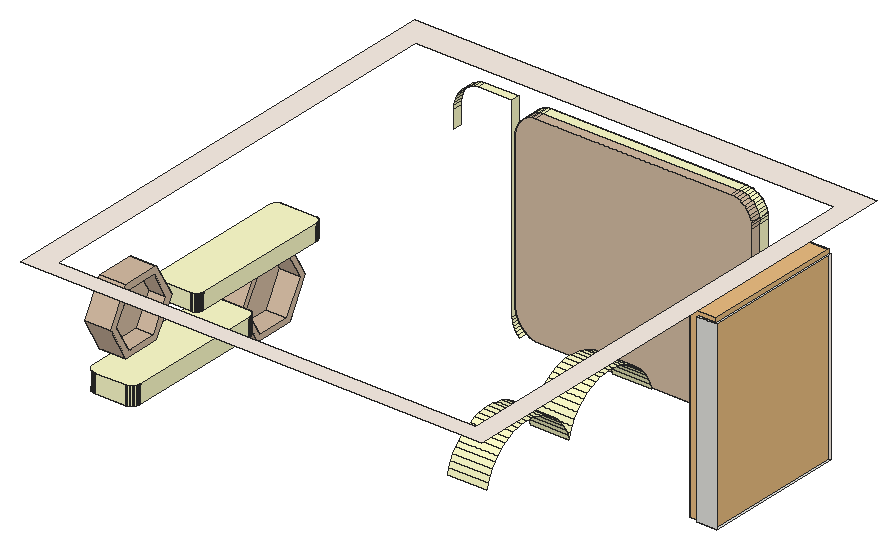
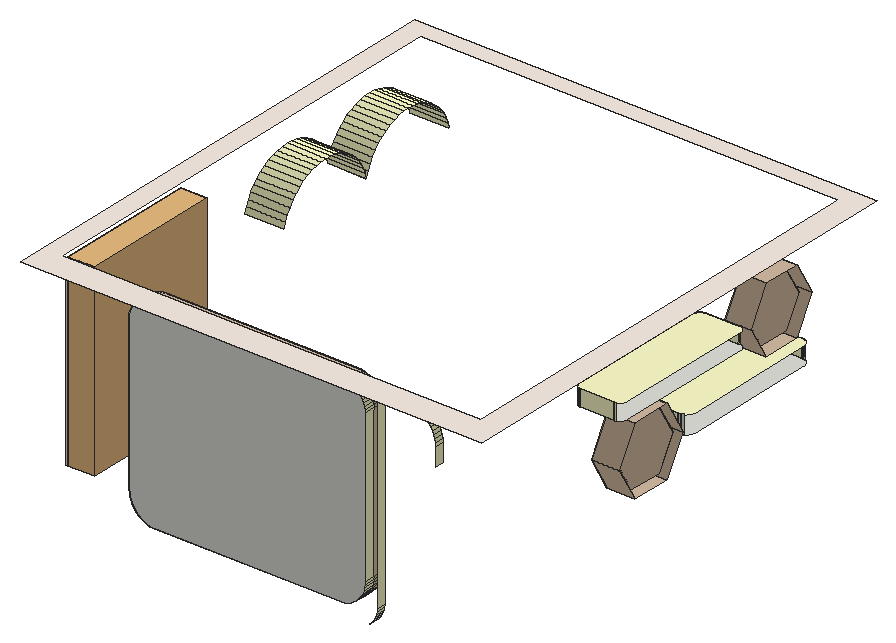
# SketchUp Ruby script. Lengths in inches.
U = 1.inch
M = Sketchup.active_model
def pt(a) = Geom::Point3d.new(a.map { |v| v * U })
def face(e, loops, mat)
  f = e.add_face(loops[0].map { |a| pt(a) })
  loops[1..].each { |l| e.add_face(l.map { |a| pt(a) }).erase! }
  f.material = f.back_material = mat if mat
  f
end
# faces: each face lists its corners as indices into pts; further lists are holes
def faces(e, pts, list, mat = nil) = list.each { |f| face(e, (f[0].is_a?(Array) ? f : [f]).map { |l| l.map { |i| pts[i] } }, mat) }
# xy, xz, yz: faces in a plane at the given z, y or x. An outline is a flat list of corners, or four numbers for a rectangle; further outlines are holes
def ring(l) = l.size == 4 ? [[l[0], l[1]], [l[2], l[1]], [l[2], l[3]], [l[0], l[3]]] : l.each_slice(2).to_a
def flat(e, list, mat, &to3) = list.each { |f| face(e, (f[0].is_a?(Array) ? f : [f]).map { |l| ring(l).map { |u, v| to3.(u, v) } }, mat) }
def xy(e, z, list, mat = nil) = flat(e, list, mat) { |x, y| [x, y, z] }
def xz(e, y, list, mat = nil) = flat(e, list, mat) { |x, z| [x, y, z] }
def yz(e, x, list, mat = nil) = flat(e, list, mat) { |y, z| [x, y, z] }
def lines(e, pts, list) = list.each { |a, b| e.add_line(pt(pts[a]), pt(pts[b])) }
# prism: a flat outline (further loops are holes) pulled along v
def prism(e, loops, v, mat = nil)
  f = face(e, loops, mat); d = Geom::Vector3d.new(v.map { |x| x * U })
  f.pushpull(f.normal.samedirection?(d) ? d.length : -d.length)
end
def box(e, o, s, mat = nil) = prism(e, [[o, [o[0] + s[0], o[1], o[2]], [o[0] + s[0], o[1] + s[1], o[2]], [o[0], o[1] + s[1], o[2]]]], [0, 0, s[2]], mat)
def at(x, y, z, deg = 0) = Geom::Transformation.translation(pt([x, y, z])) * Geom::Transformation.rotation(ORIGIN, Z_AXIS, deg.degrees)
def axes(o, x, y, z) = Geom::Transformation.new([*x, 0, *y, 0, *z, 0, *pt(o).to_a, 1])
def part(name) = M.definitions.add(name)
# library, detail: a bought-in or finely detailed component or shape, given as its bounding box
def library(name, o, s) = part(name).tap { |d| box(d.entities, o, s) }
def detail(e, o, s) = box(e.add_group.entities, o, s)
def put(e, d, t, mat = nil) = e.add_instance(d, t).tap { |i| i.material = mat if mat }
def group(e, t, mat = nil) = e.add_group.tap { |g| g.transformation = t; g.material = mat if mat }.entities
root = M.entities
M.materials.add("[0009_Linen]").color = [250, 240, 230]
M.materials.add("[Color E01]").color = [255, 255, 204]
M.materials.add("[Formica Laminate Light]").color = [213, 189, 164]
c1 = library("window",[-170.85,-38.53,47.13],[55.51,10.56,74.96])
xy(root,45.28,[[582.21,181.97,659.93,185.9375]],"[Color E01]")
xy(root,45.28,[[582.21,178,659.93,181.97]],"[Formica Laminate Light]")
xy(root,47.26,[[695.01,117.4375,702.89,174.3125]])
xy(root,67.64,[[527.89,93.09,538.95,108.9]],"[Formica Laminate Light]")
xy(root,69.47,[[530.26,94.15,538.95,107.84]],"[Formica Laminate Light]")
xy(root,78.19,[[532.01,20.91,531.51,20.9375,531.01,21.03,530.53,21.18,530.07,21.39,529.64,21.65,529.24,21.96,528.89,22.32,528.58,22.72,528.32,23.15,528.12,23.61,527.97,24.1,527.89,24.59,527.89,78.67,527.96,79.18,528.1,79.67,528.3,80.14,528.55,80.58,528.86,80.99,529.22,81.36,529.61,81.68,530.05,81.95,530.51,82.16,531,82.32,531.5,82.41,532.01,82.44,544.01,82.44,544.43,82.33,544.84,82.16,545.22,81.95,545.58,81.7,545.91,81.41,546.2,81.08,546.45,80.72,546.66,80.33,546.82,79.93,546.93,79.5,547,79.07,547.01,78.63,547.01,24.59,546.99,24.16,546.91,23.74,546.79,23.33,546.625,22.93,546.41,22.56,546.16,22.21,545.87,21.89,545.54,21.61,545.19,21.37,544.81,21.17,544.41,21.01,543.99,20.91]])
xy(root,85.38,[[532.01,20.91,543.99,20.91,544.41,21.01,544.81,21.17,545.19,21.37,545.54,21.61,545.87,21.89,546.16,22.21,546.41,22.56,546.625,22.93,546.79,23.33,546.91,23.74,546.99,24.16,547.01,24.59,547.01,78.63,547,79.07,546.93,79.5,546.82,79.93,546.66,80.33,546.45,80.72,546.2,81.08,545.91,81.41,545.58,81.7,545.22,81.95,544.84,82.16,544.43,82.33,544.01,82.44,532.01,82.44,531.5,82.41,531,82.32,530.51,82.16,530.05,81.95,529.61,81.68,529.22,81.36,528.86,80.99,528.55,80.58,528.3,80.14,528.1,79.67,527.96,79.18,527.89,78.67,527.89,24.59,527.97,24.1,528.12,23.61,528.32,23.15,528.58,22.72,528.89,22.32,529.24,21.96,529.64,21.65,530.07,21.39,530.53,21.18,531.01,21.03,531.51,20.9375]],"[Color E01]")
xy(root,89.72,[[527.89,28.21,538.2,43.44]],"[Formica Laminate Light]")
xy(root,92.04,[[531.07,29.55,538.2,42.1]],"[Formica Laminate Light]")
xy(root,93.1875,[[530.26,94.15,538.95,107.84]],"[Formica Laminate Light]")
xy(root,95.02,[[527.89,93.09,538.95,108.9]],"[Formica Laminate Light]")
xy(root,97.75,[[531.07,53.41,530.67,53.4375,530.28,53.51,529.9,53.64,529.53,53.81,529.19,54.02,528.88,54.28,528.61,54.57,528.375,54.9,528.18,55.25,528.03,55.625,527.9375,56.01,527.89,56.41,527.89,112.29,527.97,112.69,528.1,113.09,528.26,113.47,528.46,113.84,528.69,114.18,528.96,114.5,529.25,114.79,529.58,115.05,529.92,115.28,530.29,115.47,530.68,115.63,531.07,115.75,544.2,115.75,544.59,115.64,544.96,115.49,545.32,115.3,545.65,115.0625,545.95,114.8,546.22,114.5,546.46,114.17,546.65,113.8125,546.81,113.44,546.92,113.05,546.99,112.65,547.01,112.25,547.01,56.29,546.94,55.93,546.84,55.58,546.69,55.25,546.51,54.93,546.3,54.63,546.06,54.36,545.79,54.12,545.49,53.91,545.18,53.73,544.84,53.59,544.49,53.48,544.13,53.41]])
xy(root,104.19,[[531.07,53.41,544.13,53.41,544.49,53.48,544.84,53.59,545.18,53.73,545.49,53.91,545.79,54.12,546.06,54.36,546.3,54.63,546.51,54.93,546.69,55.25,546.84,55.58,546.94,55.93,547.01,56.29,547.01,112.25,546.99,112.65,546.92,113.05,546.81,113.44,546.65,113.8125,546.46,114.17,546.22,114.5,545.95,114.8,545.65,115.0625,545.32,115.3,544.96,115.49,544.59,115.64,544.2,115.75,531.07,115.75,530.68,115.63,530.29,115.47,529.92,115.28,529.58,115.05,529.25,114.79,528.96,114.5,528.69,114.18,528.46,113.84,528.26,113.47,528.1,113.09,527.97,112.69,527.89,112.29,527.89,56.41,527.9375,56.01,528.03,55.625,528.18,55.25,528.375,54.9,528.61,54.57,528.88,54.28,529.19,54.02,529.53,53.81,529.9,53.64,530.28,53.51,530.67,53.4375]],"[Color E01]")
xy(root,113.77,[[531.07,29.55,538.2,42.1]],"[Formica Laminate Light]")
xy(root,116.09,[[527.89,28.21,538.2,43.44]],"[Formica Laminate Light]")
xy(root,120.7,[[695.01,117.4375,702.89,174.3125]])
xy(root,125.3125,[[582.21,181.97,659.93,185.9375],[555.52,182.5625,569.01,185.9375]],"[Color E01]")
xy(root,125.3125,[[582.21,178,659.93,181.97]],"[Formica Laminate Light]")
xy(root,129.75,[[[518.64,0,702.89,197],[527.89,6.9375,695.01,185.9375]]],"[0009_Linen]")
xz(root,20.91,[[532.01,78.19,543.99,85.38]],"[Color E01]")
xz(root,53.41,[[531.07,97.75,544.13,104.19]],"[Color E01]")
xz(root,82.44,[[532.01,78.19,544.01,85.38]],"[Color E01]")
xz(root,115.75,[[531.07,97.75,544.2,104.19]],"[Color E01]")
xz(root,117.4375,[[695.01,47.26,702.89,120.7]])
xz(root,174.3125,[[695.01,47.26,702.89,120.7]],"[0009_Linen]")
xz(root,178,[[582.21,45.28,659.93,45.28,661.1,45.65,662.21,46.14,663.27,46.75,664.25,47.46,665.14,48.28,665.9375,49.18,666.63,50.16,667.21,51.21,667.66,52.3125,667.99,53.46,668.19,54.63,668.26,55.82,668.26,116.08,668.33,117.24,668.26,118.12,668.24,118.39,667.97,119.52,667.55,120.6,666.97,121.61,666.25,122.53,665.41,123.34,664.45,124.03,663.4,124.58,662.29,124.99,661.12,125.23,659.93,125.3125,582.21,125.3125,581.07,125.11,579.96,124.78,578.9,124.33,577.91,123.75,576.99,123.05,576.17,122.26,575.46,121.375,574.85,120.41,574.375,119.39,574.03,118.3125,573.82,117.21,573.75,116.08,573.75,55.82,573.79,54.61,573.98,53.42,574.3,52.26,574.75,51.14,575.34,50.07,576.04,49.08,576.86,48.18,577.78,47.37,578.79,46.66,579.875,46.08,581.02,45.62]],"[Formica Laminate Light]")
xz(root,185.9375,[[582.21,45.28,581.02,45.62,579.875,46.08,578.79,46.66,577.78,47.37,576.86,48.18,576.04,49.08,575.34,50.07,574.75,51.14,574.3,52.26,573.98,53.42,573.79,54.61,573.75,55.82,573.75,116.08,573.82,117.21,574.03,118.3125,574.375,119.39,574.85,120.41,575.46,121.375,576.17,122.26,576.99,123.05,577.91,123.75,578.9,124.33,579.96,124.78,581.07,125.11,582.21,125.3125,659.93,125.3125,661.12,125.23,662.29,124.99,663.4,124.58,664.45,124.03,665.41,123.34,666.25,122.53,666.97,121.61,667.55,120.6,667.97,119.52,668.24,118.39,668.26,118.12,668.33,117.24,668.26,116.08,668.26,55.82,668.19,54.63,667.99,53.46,667.66,52.3125,667.21,51.21,666.63,50.16,665.9375,49.18,665.14,48.28,664.25,47.46,663.27,46.75,662.21,46.14,661.1,45.65,659.93,45.28]])
yz(root,530.26,[[94.15,69.47,107.84,69.47,114.6875,81.33,107.84,93.1875,94.15,93.1875,87.3,81.33]],"[Formica Laminate Light]")
yz(root,531.07,[[29.55,92.04,42.1,92.04,48.375,102.9,42.1,113.77,29.55,113.77,23.28,102.9]],"[Formica Laminate Light]")
yz(root,538.2,[[[28.21,89.72,43.44,89.72,51.05,102.9,43.44,116.09,28.21,116.09,20.6,102.9],[29.55,92.04,23.28,102.9,29.55,113.77,42.1,113.77,48.375,102.9,42.1,92.04]]],"[Formica Laminate Light]")
yz(root,538.95,[[[93.09,67.64,108.9,67.64,116.8,81.33,108.9,95.02,93.09,95.02,85.1875,81.33],[94.15,69.47,87.3,81.33,94.15,93.1875,107.84,93.1875,114.6875,81.33,107.84,69.47]]],"[Formica Laminate Light]")
yz(root,545.7,[[182.5625,106.81,185.9375,113.87]],"[Color E01]")
yz(root,547.01,[[24.59,78.19,78.63,85.38],[56.29,97.75,112.25,104.19]],"[Color E01]")
yz(root,569.01,[[182.5625,47.68,185.9375,125.3125]],"[Color E01]")
yz(root,573.75,[[181.97,55.82,185.9375,116.08]],"[Color E01]")
yz(root,573.75,[[178,55.82,181.97,116.08]],"[Formica Laminate Light]")
yz(root,668.26,[[181.97,55.82,185.9375,116.08]],"[Color E01]")
yz(root,668.26,[[178,55.82,181.97,116.08]],"[Formica Laminate Light]")
p = [[571.35,185.9375,42.03],[571.35,182.5625,42.03],[572.14,182.5625,41.34],[572.14,185.9375,41.34],[570.66,185.9375,42.8125],[570.66,182.5625,42.8125],
  [570.08,185.9375,43.68],[570.08,182.5625,43.68],[569.62,185.9375,44.62],[569.62,182.5625,44.62],[569.28,185.9375,45.61],[569.28,182.5625,45.61],
  [581.02,178,45.62],[581.02,181.97,45.62],[582.21,181.97,45.28],[582.21,178,45.28],[659.93,178,45.28],[659.93,181.97,45.28],
  [661.1,181.97,45.65],[661.1,178,45.65],[582.21,185.9375,45.28],[581.02,185.9375,45.62],[661.1,185.9375,45.65],[659.93,185.9375,45.28],
  [579.875,178,46.08],[579.875,181.97,46.08],[579.875,185.9375,46.08],[569.08,185.9375,46.64],[569.08,182.5625,46.64],[662.21,181.97,46.14],
  [662.21,178,46.14],[662.21,185.9375,46.14],[578.79,178,46.66],[578.79,181.97,46.66],[663.27,181.97,46.75],[663.27,178,46.75],
  [578.79,185.9375,46.66],[663.27,185.9375,46.75],[569.01,185.9375,47.68],[569.01,182.5625,47.68],[577.78,178,47.37],[577.78,181.97,47.37],
  [664.25,181.97,47.46],[664.25,178,47.46],[577.78,185.9375,47.37],[664.25,185.9375,47.46],[576.86,178,48.18],[576.86,181.97,48.18],
  [576.86,185.9375,48.18],[665.14,181.97,48.28],[665.14,178,48.28],[665.14,185.9375,48.28],[576.04,178,49.08],[576.04,181.97,49.08],
  [576.04,185.9375,49.08],[665.9375,181.97,49.18],[665.9375,178,49.18],[665.9375,185.9375,49.18],[575.34,178,50.07],[575.34,181.97,50.07],
  [575.34,185.9375,50.07],[666.63,181.97,50.16],[666.63,178,50.16],[666.63,185.9375,50.16],[574.75,178,51.14],[574.75,181.97,51.14],
  [574.75,185.9375,51.14],[667.21,181.97,51.21],[667.21,178,51.21],[667.21,185.9375,51.21],[574.3,178,52.26],[574.3,181.97,52.26],
  [574.3,185.9375,52.26],[667.66,181.97,52.3125],[667.66,178,52.3125],[667.66,185.9375,52.3125],[573.98,178,53.42],[573.98,181.97,53.42],
  [667.99,181.97,53.46],[667.99,178,53.46],[573.98,185.9375,53.42],[667.99,185.9375,53.46],[573.79,178,54.61],[573.79,181.97,54.61],
  [573.79,185.9375,54.61],[668.19,181.97,54.63],[668.19,178,54.63],[668.19,185.9375,54.63],[573.75,178,55.82],[573.75,181.97,55.82],
  [668.26,181.97,55.82],[668.26,178,55.82],[573.75,185.9375,55.82],[668.26,185.9375,55.82],[527.89,85.1875,81.33],[527.89,93.09,67.64],
  [538.95,93.09,67.64],[538.95,85.1875,81.33],[527.89,108.9,67.64],[527.89,116.8,81.33],[538.95,116.8,81.33],[538.95,108.9,67.64],
  [538.95,87.3,81.33],[538.95,94.15,69.47],[530.26,94.15,69.47],[530.26,87.3,81.33],[538.95,107.84,69.47],[538.95,114.6875,81.33],
  [530.26,114.6875,81.33],[530.26,107.84,69.47],[531.51,20.9375,85.38],[531.01,21.03,85.38],[531.01,21.03,78.19],[531.51,20.9375,78.19],
  [532.01,20.91,85.38],[532.01,20.91,78.19],[544.41,21.01,85.38],[543.99,20.91,85.38],[543.99,20.91,78.19],[544.41,21.01,78.19],
  [530.53,21.18,85.38],[530.53,21.18,78.19],[544.81,21.17,85.38],[544.81,21.17,78.19],[530.07,21.39,85.38],[530.07,21.39,78.19],
  [545.19,21.37,85.38],[545.19,21.37,78.19],[545.54,21.61,85.38],[545.54,21.61,78.19],[545.87,21.89,85.38],[545.87,21.89,78.19],
  [546.16,22.21,85.38],[546.16,22.21,78.19],[546.41,22.56,85.38],[546.41,22.56,78.19],[546.625,22.93,85.38],[546.625,22.93,78.19],
  [546.79,23.33,85.38],[546.79,23.33,78.19],[546.91,23.74,85.38],[546.91,23.74,78.19],[546.99,24.16,85.38],[546.99,24.16,78.19],
  [547.01,24.59,85.38],[547.01,24.59,78.19],[547,79.07,85.38],[547.01,78.63,85.38],[547.01,78.63,78.19],[547,79.07,78.19],
  [546.93,79.5,85.38],[546.93,79.5,78.19],[546.82,79.93,85.38],[546.82,79.93,78.19],[546.66,80.33,85.38],[546.66,80.33,78.19],
  [546.45,80.72,85.38],[546.45,80.72,78.19],[546.2,81.08,85.38],[546.2,81.08,78.19],[545.91,81.41,85.38],[545.91,81.41,78.19],
  [545.58,81.7,85.38],[545.58,81.7,78.19],[545.22,81.95,85.38],[545.22,81.95,78.19],[530.05,81.95,85.38],[530.51,82.16,85.38],
  [530.51,82.16,78.19],[530.05,81.95,78.19],[544.84,82.16,85.38],[544.84,82.16,78.19],[531,82.32,85.38],[531,82.32,78.19],
  [544.43,82.33,85.38],[544.43,82.33,78.19],[531.5,82.41,85.38],[531.5,82.41,78.19],[544.01,82.44,85.38],[544.01,82.44,78.19],
  [532.01,82.44,85.38],[532.01,82.44,78.19],[527.89,93.09,95.02],[538.95,93.09,95.02],[538.95,94.15,93.1875],[530.26,94.15,93.1875],
  [538.95,107.84,93.1875],[530.26,107.84,93.1875],[527.89,108.9,95.02],[538.95,108.9,95.02],[527.89,20.6,102.9],[527.89,28.21,89.72],
  [538.2,28.21,89.72],[538.2,20.6,102.9],[527.89,43.44,89.72],[527.89,51.05,102.9],[538.2,51.05,102.9],[538.2,43.44,89.72],
  [538.2,23.28,102.9],[538.2,29.55,92.04],[531.07,29.55,92.04],[531.07,23.28,102.9],[538.2,42.1,92.04],[538.2,48.375,102.9],
  [531.07,48.375,102.9],[531.07,42.1,92.04],[530.67,53.4375,104.19],[530.28,53.51,104.19],[530.28,53.51,97.75],[530.67,53.4375,97.75],
  [531.07,53.41,104.19],[531.07,53.41,97.75],[544.49,53.48,104.19],[544.13,53.41,104.19],[544.13,53.41,97.75],[544.49,53.48,97.75],
  [544.84,53.59,104.19],[544.84,53.59,97.75],[545.18,53.73,104.19],[545.18,53.73,97.75],[545.49,53.91,104.19],[545.49,53.91,97.75],
  [545.79,54.12,104.19],[545.79,54.12,97.75],[546.06,54.36,104.19],[546.06,54.36,97.75],[546.3,54.63,104.19],[546.3,54.63,97.75],
  [546.51,54.93,104.19],[546.51,54.93,97.75],[546.69,55.25,104.19],[546.69,55.25,97.75],[546.84,55.58,104.19],[546.84,55.58,97.75],
  [546.94,55.93,104.19],[546.94,55.93,97.75],[547.01,56.29,104.19],[547.01,56.29,97.75],[546.99,112.65,104.19],[547.01,112.25,104.19],
  [547.01,112.25,97.75],[546.99,112.65,97.75],[546.92,113.05,104.19],[546.92,113.05,97.75],[546.81,113.44,104.19],[546.81,113.44,97.75],
  [546.65,113.8125,104.19],[546.65,113.8125,97.75],[546.46,114.17,104.19],[546.46,114.17,97.75],[546.22,114.5,104.19],[546.22,114.5,97.75],
  [545.95,114.8,104.19],[545.95,114.8,97.75],[545.65,115.0625,104.19],[545.65,115.0625,97.75],[545.32,115.3,104.19],[545.32,115.3,97.75],
  [544.96,115.49,104.19],[544.96,115.49,97.75],[530.29,115.47,104.19],[530.68,115.63,104.19],[530.68,115.63,97.75],[530.29,115.47,97.75],
  [544.59,115.64,104.19],[544.59,115.64,97.75],[531.07,115.75,104.19],[531.07,115.75,97.75],[544.2,115.75,104.19],[544.2,115.75,97.75],
  [527.89,28.21,116.09],[538.2,28.21,116.09],[538.2,29.55,113.77],[531.07,29.55,113.77],[538.2,42.1,113.77],[531.07,42.1,113.77],
  [527.89,43.44,116.09],[538.2,43.44,116.09],[695.01,12.1875,104.7],[695.01,12.84,106.92],[679.64,12.84,106.92],[679.64,12.1875,104.7],
  [695.01,52.625,106.94],[695.01,53.375,104.7],[679.64,53.375,104.7],[679.64,52.625,106.94],[695.01,54.03,106.92],[679.64,54.03,106.92],
  [695.01,93.8125,106.94],[695.01,94.5625,104.7],[679.64,94.5625,104.7],[679.64,93.8125,106.94],[695.01,13.74,109.06],[679.64,13.74,109.06],
  [695.01,51.64,109.09],[679.64,51.64,109.09],[695.01,54.93,109.06],[679.64,54.93,109.06],[695.01,92.83,109.09],[679.64,92.83,109.09],
  [695.01,14.87,111.08],[679.64,14.87,111.08],[695.01,50.42,111.11],[679.64,50.42,111.11],[695.01,56.06,111.08],[679.64,56.06,111.08],
  [695.01,91.61,111.11],[679.64,91.61,111.11],[695.01,16.22,112.96],[679.64,16.22,112.96],[695.01,49,113],[679.64,49,113],
  [695.01,57.4,112.96],[679.64,57.4,112.96],[695.01,90.18,113],[679.64,90.18,113],[695.01,17.76,114.68],[679.64,17.76,114.68],
  [695.01,47.375,114.71],[679.64,47.375,114.71],[695.01,58.95,114.68],[679.64,58.95,114.68],[695.01,88.5625,114.71],[679.64,88.5625,114.71],
  [545.7,185.9375,113.87],[545.7,182.5625,113.87],[545.78,182.5625,115.23],[545.78,185.9375,115.23],[695.01,19.5,116.22],[679.64,19.5,116.22],
  [695.01,45.58,116.24],[679.64,45.58,116.24],[695.01,60.68,116.22],[679.64,60.68,116.22],[695.01,86.76,116.24],[679.64,86.76,116.24],
  [546.02,182.5625,116.58],[546.02,185.9375,116.58],[573.82,178,117.21],[573.82,181.97,117.21],[573.75,181.97,116.08],[573.75,178,116.08],
  [668.26,178,116.08],[668.26,181.97,116.08],[668.33,181.97,117.24],[668.33,178,117.24],[573.75,185.9375,116.08],[573.82,185.9375,117.21],
  [668.33,185.9375,117.24],[668.26,185.9375,116.08],[695.01,21.39,117.55],[679.64,21.39,117.55],[695.01,43.62,117.57],[679.64,43.62,117.57],
  [695.01,62.57,117.55],[679.64,62.57,117.55],[695.01,84.81,117.57],[679.64,84.81,117.57],[546.42,182.5625,117.89],[546.42,185.9375,117.89],
  [574.03,178,118.3125],[574.03,181.97,118.3125],[668.26,181.97,118.12],[668.26,178,118.12],[574.03,185.9375,118.3125],[668.26,185.9375,118.12],
  [695.01,23.42,118.66],[679.64,23.42,118.66],[695.01,64.6,118.66],[679.64,64.6,118.66],[695.01,41.54,118.68],[679.64,41.54,118.68],
  [695.01,82.72,118.68],[679.64,82.72,118.68],[546.97,182.5625,119.14],[546.97,185.9375,119.14],[668.24,181.97,118.39],[668.24,178,118.39],
  [668.24,185.9375,118.39],[574.375,178,119.39],[574.375,181.97,119.39],[574.375,185.9375,119.39],[667.97,181.97,119.52],[667.97,178,119.52],
  [667.97,185.9375,119.52],[695.01,25.56,119.55],[679.64,25.56,119.55],[695.01,39.34,119.56],[679.64,39.34,119.56],[695.01,66.74,119.55],
  [679.64,66.74,119.55],[695.01,80.53,119.56],[679.64,80.53,119.56],[547.66,182.5625,120.32],[547.66,185.9375,120.32],[574.85,178,120.41],
  [574.85,181.97,120.41],[574.85,185.9375,120.41],[695.01,27.78,120.19],[679.64,27.78,120.19],[695.01,68.97,120.19],[679.64,68.97,120.19],
  [667.55,181.97,120.6],[667.55,178,120.6],[667.55,185.9375,120.6],[695.01,37.07,120.1875],[679.64,37.07,120.1875],[695.01,78.25,120.1875],
  [679.64,78.25,120.1875],[695.01,30.0625,120.57],[679.64,30.0625,120.57],[695.01,34.73,120.57],[679.64,34.73,120.57],[695.01,71.25,120.57],
  [679.64,71.25,120.57],[695.01,75.92,120.57],[679.64,75.92,120.57],[548.49,182.5625,121.41],[548.49,185.9375,121.41],[575.46,178,121.375],
  [575.46,181.97,121.375],[575.46,185.9375,121.375],[695.01,32.375,120.7],[679.64,32.375,120.7],[679.64,32.36,120.7],[695.01,73.5625,120.7],
  [679.64,73.5625,120.7],[666.97,181.97,121.61],[666.97,178,121.61],[666.97,185.9375,121.61],[576.17,178,122.26],[576.17,181.97,122.26],
  [576.17,185.9375,122.26],[549.4375,182.5625,122.39],[549.4375,185.9375,122.39],[666.25,181.97,122.53],[666.25,178,122.53],[666.25,185.9375,122.53],
  [576.99,178,123.05],[576.99,181.97,123.05],[576.99,185.9375,123.05],[550.5,182.5625,123.25],[550.5,185.9375,123.25],[665.41,181.97,123.34],
  [665.41,178,123.34],[665.41,185.9375,123.34],[577.91,178,123.75],[577.91,181.97,123.75],[577.91,185.9375,123.75],[664.45,181.97,124.03],
  [664.45,178,124.03],[664.45,185.9375,124.03],[551.65,182.5625,123.99],[551.65,185.9375,123.99],[578.9,178,124.33],[578.9,181.97,124.33],
  [578.9,185.9375,124.33],[663.4,181.97,124.58],[663.4,178,124.58],[663.4,185.9375,124.58],[552.89,182.5625,124.58],[552.89,185.9375,124.58],
  [579.96,178,124.78],[579.96,181.97,124.78],[579.96,185.9375,124.78],[662.29,181.97,124.99],[662.29,178,124.99],[662.29,185.9375,124.99],
  [554.18,182.5625,125.02],[554.18,185.9375,125.02],[581.07,178,125.11],[581.07,181.97,125.11],[581.07,185.9375,125.11],[661.12,181.97,125.23],
  [661.12,178,125.23],[661.12,185.9375,125.23],[555.52,182.5625,125.3125],[555.52,185.9375,125.3125],[582.21,178,125.3125],[582.21,181.97,125.3125],
  [582.21,185.9375,125.3125],[659.93,181.97,125.3125],[659.93,178,125.3125],[659.93,185.9375,125.3125],[679.64,32.36,120.96]]
faces(root,p,[[0,1,2,3],[4,5,1,0],[6,7,5,4],[8,9,7,6],[10,11,9,8],[20,14,13,21],[22,18,17,23],[21,13,25,26],
  [27,28,11,10],[31,29,18,22],[26,25,33,36],[37,34,29,31],[38,39,28,27],[36,33,41,44],[45,42,34,37],[44,41,47,48],
  [51,49,42,45],[48,47,53,54],[57,55,49,51],[54,53,59,60],[63,61,55,57],[60,59,65,66],[69,67,61,63],[66,65,71,72],
  [75,73,67,69],[72,71,77,80],[81,78,73,75],[80,77,83,84],[87,85,78,81],[84,83,89,92],[93,90,85,87],[110,111,112,113],
  [114,110,113,115],[116,117,118,119],[111,120,121,112],[122,116,119,123],[120,124,125,121],[126,122,123,127],[128,126,127,129],[130,128,129,131],
  [132,130,131,133],[134,132,133,135],[136,134,135,137],[138,136,137,139],[140,138,139,141],[142,140,141,143],[144,142,143,145],[146,147,148,149],
  [150,146,149,151],[152,150,151,153],[154,152,153,155],[156,154,155,157],[158,156,157,159],[160,158,159,161],[162,160,161,163],[164,162,163,165],
  [170,164,165,171],[174,170,171,175],[178,174,175,179],[206,207,208,209],[210,206,209,211],[212,213,214,215],[216,212,215,217],[218,216,217,219],
  [220,218,219,221],[222,220,221,223],[224,222,223,225],[226,224,225,227],[228,226,227,229],[230,228,229,231],[232,230,231,233],[234,232,233,235],
  [236,234,235,237],[238,239,240,241],[242,238,241,243],[244,242,243,245],[246,244,245,247],[248,246,247,249],[250,248,249,251],[252,250,251,253],
  [254,252,253,255],[256,254,255,257],[258,256,257,259],[260,261,262,263],[264,258,259,265],[261,266,267,262],[268,264,265,269],[278,279,280,281],
  [282,283,284,285],[283,286,287,284],[288,289,290,291],[279,292,293,280],[294,282,285,295],[286,296,297,287],[298,288,291,299],[292,300,301,293],
  [302,294,295,303],[296,304,305,297],[306,298,299,307],[300,308,309,301],[310,302,303,311],[304,312,313,305],[314,306,307,315],[308,316,317,309],
  [318,310,311,319],[312,320,321,313],[322,314,315,323],[324,325,326,327],[316,328,329,317],[330,318,319,331],[320,332,333,321],[334,322,323,335],
  [327,326,336,337],[346,340,339,347],[348,344,343,349],[328,350,351,329],[352,330,331,353],[332,354,355,333],[356,334,335,357],[337,336,358,359],
  [347,339,361,364],[365,362,344,348],[350,366,367,351],[354,368,369,355],[370,352,353,371],[372,356,357,373],[359,358,374,375],[378,376,362,365],
  [364,361,380,381],[384,382,376,378],[366,385,386,367],[387,370,371,388],[368,389,390,369],[391,372,373,392],[375,374,393,394],[381,380,396,397],
  [385,398,399,386],[389,400,401,390],[404,402,382,384],[405,387,388,406],[407,391,392,408],[398,409,410,399],[411,405,406,412],[400,413,414,401],
  [415,407,408,416],[394,393,417,418],[397,396,420,421],[409,422,423,424,410],[422,411,412,423],[413,425,426,414],[425,415,416,426],[429,427,402,404],
  [421,420,431,432],[418,417,433,434],[437,435,427,429],[432,431,439,440],[434,433,441,442],[445,443,435,437],[440,439,447,448],[451,449,443,445],
  [442,441,452,453],[448,447,455,456],[459,457,449,451],[453,452,460,461],[456,455,463,464],[467,465,457,459],[461,460,468,469],[464,463,471,472],
  [475,473,465,467],[469,468,476,477],[472,471,479,480],[483,481,473,475]],"[Color E01]")
faces(root,p,[[12,13,14,15],[16,17,18,19],[24,25,13,12],[19,18,29,30],[32,33,25,24],[30,29,34,35],[40,41,33,32],[35,34,42,43],
  [46,47,41,40],[43,42,49,50],[52,53,47,46],[50,49,55,56],[58,59,53,52],[56,55,61,62],[64,65,59,58],[62,61,67,68],
  [70,71,65,64],[68,67,73,74],[76,77,71,70],[74,73,78,79],[82,83,77,76],[79,78,85,86],[88,89,83,82],[86,85,90,91],
  [94,95,96,97],[98,99,100,101],[102,103,104,105],[106,107,108,109],[182,94,97,183],[184,102,105,185],[107,186,187,108],[99,188,189,100],
  [190,191,192,193],[194,195,196,197],[198,199,200,201],[202,203,204,205],[270,190,193,271],[272,198,201,273],[203,274,275,204],[195,276,277,196],
  [338,339,340,341],[342,343,344,345],[360,361,339,338],[345,344,362,363],[363,362,376,377],[379,380,361,360],[377,376,382,383],[395,396,380,379],
  [383,382,402,403],[419,420,396,395],[403,402,427,428],[430,431,420,419],[428,427,435,436],[438,439,431,430],[436,435,443,444],[446,447,439,438],
  [444,443,449,450],[454,455,447,446],[450,449,457,458],[462,463,455,454],[458,457,465,466],[470,471,463,462],[466,465,473,474],[478,479,471,470],
  [474,473,481,482]],"[Formica Laminate Light]")
faces(root,p,[[166,167,168,169],[167,172,173,168],[172,176,177,173],[176,180,181,177]])
lines(root,p,[[484,424]])
put(root,c1,axes([663.3125,290.86,0],[0,1.01,0],[-1,0,0],[0,0,1]))
